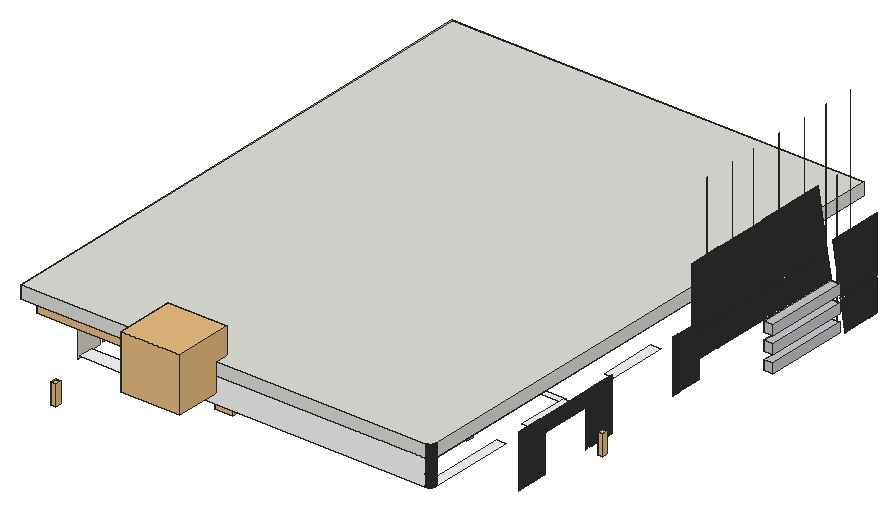
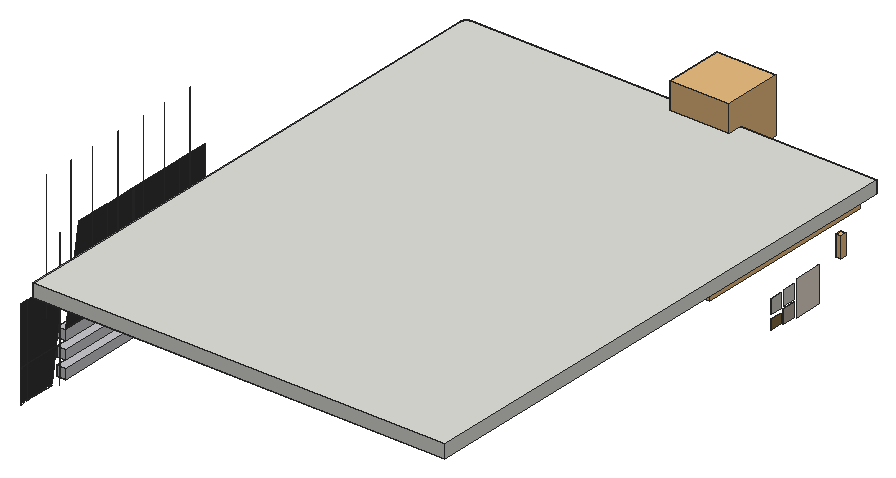
# SketchUp Ruby script. Lengths in inches.
U = 1.inch
M = Sketchup.active_model
def pt(a) = Geom::Point3d.new(a.map { |v| v * U })
def face(e, loops, mat)
  f = e.add_face(loops[0].map { |a| pt(a) })
  loops[1..].each { |l| e.add_face(l.map { |a| pt(a) }).erase! }
  f.material = f.back_material = mat if mat
  f
end
# faces: each face lists its corners as indices into pts; further lists are holes
def faces(e, pts, list, mat = nil) = list.each { |f| face(e, (f[0].is_a?(Array) ? f : [f]).map { |l| l.map { |i| pts[i] } }, mat) }
# xy, xz, yz: faces in a plane at the given z, y or x. An outline is a flat list of corners, or four numbers for a rectangle; further outlines are holes
def ring(l) = l.size == 4 ? [[l[0], l[1]], [l[2], l[1]], [l[2], l[3]], [l[0], l[3]]] : l.each_slice(2).to_a
def flat(e, list, mat, &to3) = list.each { |f| face(e, (f[0].is_a?(Array) ? f : [f]).map { |l| ring(l).map { |u, v| to3.(u, v) } }, mat) }
def xy(e, z, list, mat = nil) = flat(e, list, mat) { |x, y| [x, y, z] }
def xz(e, y, list, mat = nil) = flat(e, list, mat) { |x, z| [x, y, z] }
def yz(e, x, list, mat = nil) = flat(e, list, mat) { |y, z| [x, y, z] }
def lines(e, pts, list) = list.each { |a, b| e.add_line(pt(pts[a]), pt(pts[b])) }
# prism: a flat outline (further loops are holes) pulled along v
def prism(e, loops, v, mat = nil)
  f = face(e, loops, mat); d = Geom::Vector3d.new(v.map { |x| x * U })
  f.pushpull(f.normal.samedirection?(d) ? d.length : -d.length)
end
def box(e, o, s, mat = nil) = prism(e, [[o, [o[0] + s[0], o[1], o[2]], [o[0] + s[0], o[1] + s[1], o[2]], [o[0], o[1] + s[1], o[2]]]], [0, 0, s[2]], mat)
def at(x, y, z, deg = 0) = Geom::Transformation.translation(pt([x, y, z])) * Geom::Transformation.rotation(ORIGIN, Z_AXIS, deg.degrees)
def axes(o, x, y, z) = Geom::Transformation.new([*x, 0, *y, 0, *z, 0, *pt(o).to_a, 1])
def part(name) = M.definitions.add(name)
# library, detail: a bought-in or finely detailed component or shape, given as its bounding box
def library(name, o, s) = part(name).tap { |d| box(d.entities, o, s) }
def detail(e, o, s) = box(e.add_group.entities, o, s)
def put(e, d, t, mat = nil) = e.add_instance(d, t).tap { |i| i.material = mat if mat }
def group(e, t, mat = nil) = e.add_group.tap { |g| g.transformation = t; g.material = mat if mat }.entities
root = M.entities
M.materials.add("1513 AP K108 Rose Silver-N").color = [202, 201, 205]
M.materials.add("Laura_Hair").color = [160, 135, 94]
M.materials.add("Screenshot 2024-11-21 122829").color = [225, 216, 203]
M.materials.add("Screenshot 2024-11-21 123111").color = [210, 207, 202]
M.materials.add("Screenshot 2024-11-21 123347").color = [204, 201, 193]
M.materials.add("Screenshot 2024-11-21 123542").color = [178, 168, 157]
M.materials.add("Screenshot 2024-11-21 123654").color = [134, 109, 66]
M.materials.add("[0043_SaddleBrown]1").color = [139, 97, 33]
M.materials.add("[0047_Khaki]").color = [240, 230, 140]
M.materials.add("[0135_DarkGray]1").color = [81, 81, 81]
M.materials.add("[0136_Charcoal]").color = [35, 35, 35]
M.materials.add("[0137_Black]").color = [0, 0, 0]
M.materials.add("[Color D01]").color = [255, 242, 204]
M.materials.add("[Granite Dark Gray]").color = [51, 50, 50]
M.materials.add("[Quartz Light Grey]").color = [251, 251, 252]
c1 = library("UPLOAD",[122.71,32.39,0],[21.72,7.04,54.93])
c2 = part("4")
box(c2.entities,[0,-36,0],[9,78.24,9])
c3 = library("alu art",[7.69,0,0],[1.58,66.37,36.6])
c4 = part("Component\#78")
xy(c4.entities,0,[[0,0,6,9]],"Screenshot 2024-11-21 123347")
xy(c4.entities,1.5,[[0,0,6,9]],"Screenshot 2024-11-21 123347")
xz(c4.entities,0,[[0,0,6,1.5]],"[0047_Khaki]")
xz(c4.entities,9,[[0,0,6,1.5]],"[0047_Khaki]")
yz(c4.entities,0,[[0,0,9,1.5]],"[0047_Khaki]")
yz(c4.entities,6,[[0,0,9,1.5]],"[0047_Khaki]")
c5 = part("Component\#77")
xy(c5.entities,0,[[0,0,6,8]],"Screenshot 2024-11-21 123111")
xy(c5.entities,0.375,[[0,0,6,8]],"Screenshot 2024-11-21 123111")
xz(c5.entities,0,[[0,0,6,0.375]],"[0136_Charcoal]")
xz(c5.entities,8,[[0,0,6,0.375]],"[0136_Charcoal]")
yz(c5.entities,0,[[0,0,8,0.375]],"[0136_Charcoal]")
yz(c5.entities,6,[[0,0,8,0.375]],"[0136_Charcoal]")
c6 = part("Component\#76")
xy(c6.entities,0,[[0,0,24,36]],"Screenshot 2024-11-21 122829")
xy(c6.entities,0.7,[[0,0,24,36]],"Screenshot 2024-11-21 122829")
xz(c6.entities,0,[[0,0,24,0.7]],"[0135_DarkGray]1")
xz(c6.entities,36,[[0,0,24,0.7]],"[0135_DarkGray]1")
yz(c6.entities,0,[[0,0,36,0.7]],"[0135_DarkGray]1")
yz(c6.entities,24,[[0,0,36,0.7]],"[0135_DarkGray]1")
c7 = part("Component\#80")
xy(c7.entities,0,[[0,0,10,8]],"Screenshot 2024-11-21 123654")
xy(c7.entities,1.5,[[0,0,10,8]],"Screenshot 2024-11-21 123654")
xz(c7.entities,0,[[0,0,10,1.5]],"[0043_SaddleBrown]1")
xz(c7.entities,8,[[0,0,10,1.5]],"[0043_SaddleBrown]1")
yz(c7.entities,0,[[0,0,8,1.5]],"[0043_SaddleBrown]1")
yz(c7.entities,10,[[0,0,8,1.5]],"[0043_SaddleBrown]1")
c8 = part("Component\#79")
xy(c8.entities,0,[[0,0,6,6]],"Screenshot 2024-11-21 123542")
xy(c8.entities,1.5,[[0,0,6,6]],"Screenshot 2024-11-21 123542")
xz(c8.entities,0,[[0,0,6,1.5]],"[0137_Black]")
xz(c8.entities,6,[[0,0,6,1.5]],"[0137_Black]")
yz(c8.entities,0,[[0,0,6,1.5]],"[0137_Black]")
yz(c8.entities,6,[[0,0,6,1.5]],"[0137_Black]")
c9 = part("wallart")
g1 = group(c9.entities,at(0,0,0))
put(g1,c4,axes([44.59,0,15.65],[1.7388,0,0],[0,0,1.4322],[0,-0.42,0]))
put(g1,c5,axes([29.35,0,16.47],[1.9152,0,0],[0,0,1.68],[0,-1.68,0]))
put(g1,c6,axes([0,0,0],[1.06957,0,0],[0,0,0.8988],[0,-0.8988,0]),"[0136_Charcoal]")
put(g1,c7,axes([45.17,0,2.94],[1.05,0,0],[0,0,1.1046],[0,-0.42,0]))
put(g1,c8,axes([28.96,0,1.29],[2.0328,0,0],[0,0,2.1],[0,-0.42,0]))
c10 = library("WALL LIGHT 69",[4.19,4.05,-9.63],[4.61,5.7,18.83])
c11 = library("Group\#103",[0,0,0],[31.5,31.5,74.4])
c12 = library("Group\#95",[0,0,0],[31.5,31.5,74.4])
c13 = library("Group\#83",[0,0,0],[31.5,31.5,74.4])
c14 = library("Group\#86",[0,0,0],[31.5,31.5,74.4])
c15 = library("Group\#85",[0,0,0],[31.5,31.5,74.4])
c16 = library("Group\#118",[0,0,0],[31.5,31.5,74.4])
c17 = part("Plant Wall Art")
g2 = group(c17.entities,at(1.72,0.59,0))
xy(g2,0,[[0,-0.59,13.78,0]],"Laura_Hair")
xy(g2,0.39,[[0.39,-0.59,13.39,-0.39]],"Laura_Hair")
xy(g2,19.29,[[0.39,-0.59,13.39,-0.39]],"Laura_Hair")
xy(g2,19.69,[[0,-0.59,13.78,0]],"Laura_Hair")
xz(g2,-0.59,[[[0,0,13.78,19.69],[0.39,0.39,13.39,19.29]]],"Laura_Hair")
xz(g2,0,[[0,0,13.78,19.69]],"Laura_Hair")
yz(g2,0,[[-0.59,0,0,19.69]],"Laura_Hair")
yz(g2,0.39,[[-0.59,0.39,-0.39,19.29]],"Laura_Hair")
yz(g2,13.39,[[-0.59,0.39,-0.39,19.29]],"Laura_Hair")
yz(g2,13.78,[[-0.59,0,0,19.69]],"Laura_Hair")
p = [[13.39,0,0.39],[13.39,-0.39,0.39],[13.39,0,19.29],[13.39,-0.39,19.29],[0.39,0,0.39],[0.39,-0.39,0.39],
  [0.39,0,19.29],[0.39,-0.39,19.29]]
lines(g2,p,[[0,1],[2,3],[4,5],[6,7]])
g3 = group(c17.entities,at(19.43,0.59,0))
xy(g3,0,[[0,-0.59,13.78,0]],"Laura_Hair")
xy(g3,0.39,[[0.39,-0.59,13.39,-0.39]],"Laura_Hair")
xy(g3,19.29,[[0.39,-0.59,13.39,-0.39]],"Laura_Hair")
xy(g3,19.69,[[0,-0.59,13.78,0]],"Laura_Hair")
xz(g3,-0.59,[[[0,0,13.78,19.69],[0.39,0.39,13.39,19.29]]],"Laura_Hair")
xz(g3,0,[[0,0,13.78,19.69]],"Laura_Hair")
yz(g3,0,[[-0.59,0,0,19.69]],"Laura_Hair")
yz(g3,0.39,[[-0.59,0.39,-0.39,19.29]],"Laura_Hair")
yz(g3,13.39,[[-0.59,0.39,-0.39,19.29]],"Laura_Hair")
yz(g3,13.78,[[-0.59,0,0,19.69]],"Laura_Hair")
p = [[13.39,0,0.39],[13.39,-0.39,0.39],[13.39,0,19.29],[13.39,-0.39,19.29],[0.39,0,0.39],[0.39,-0.39,0.39],
  [0.39,0,19.29],[0.39,-0.39,19.29]]
lines(g3,p,[[0,1],[2,3],[4,5],[6,7]])
g4 = group(c17.entities,at(37.15,0.59,0))
xy(g4,0,[[0,-0.59,13.78,0]],"Laura_Hair")
xy(g4,0.39,[[0.39,-0.59,13.39,-0.39]],"Laura_Hair")
xy(g4,19.29,[[0.39,-0.59,13.39,-0.39]],"Laura_Hair")
xy(g4,19.69,[[0,-0.59,13.78,0]],"Laura_Hair")
xz(g4,-0.59,[[[0,0,13.78,19.69],[0.39,0.39,13.39,19.29]]],"Laura_Hair")
xz(g4,0,[[0,0,13.78,19.69]],"Laura_Hair")
yz(g4,0,[[-0.59,0,0,19.69]],"Laura_Hair")
yz(g4,0.39,[[-0.59,0.39,-0.39,19.29]],"Laura_Hair")
yz(g4,13.39,[[-0.59,0.39,-0.39,19.29]],"Laura_Hair")
yz(g4,13.78,[[-0.59,0,0,19.69]],"Laura_Hair")
p = [[13.39,0,0.39],[13.39,-0.39,0.39],[13.39,0,19.29],[13.39,-0.39,19.29],[0.39,0,0.39],[0.39,-0.39,0.39],
  [0.39,0,19.29],[0.39,-0.39,19.29]]
lines(g4,p,[[0,1],[2,3],[4,5],[6,7]])
c18 = library("Potted trailing plant",[-13.52,-13.75,-7.41],[40.56,40.5625,37.31])
c19 = library("Group\#499",[0,24,0],[134.36,119.61,16.18])
xy(root,164,[[443.875,563.39,444,591],[443.875,592,444,600]],"[Granite Dark Gray]")
xy(root,165,[[443.875,563.22,444,591],[443.875,592,444,600]],"[Granite Dark Gray]")
xy(root,194,[[443.875,558.17,444,591],[443.875,592,444,600]],"[Granite Dark Gray]")
xy(root,195,[[443.875,558,444,591],[443.875,592,444,600]],"[Granite Dark Gray]")
xy(root,199,[[443.875,183,444,207],[443.875,208,444,213],[443.875,261,444,267],[443.875,268,444,291],[443.875,363,444,369],
  [443.875,370,444,393]],"[Granite Dark Gray]")
xy(root,200,[[443.875,183,444,207],[443.875,208,444,213],[443.875,261,444,267],[443.875,268,444,291],[443.875,363,444,369],
  [443.875,370,444,393]],"[Granite Dark Gray]")
xy(root,210,[[436.875,393,437,423],[436.875,424,437,477],[436.875,478,437,507],[436.875,508,437,555.39]],"[Granite Dark Gray]")
xy(root,211,[[436.875,393,437,423],[436.875,424,437,477],[436.875,478,437,507],[436.875,508,437,555.22]],"[Granite Dark Gray]")
xy(root,222,[[351,273,411,279]],"[Quartz Light Grey]")
xy(root,234,[[432,213,444,261],[436.875,393,437,423],[436.875,424,437,477],[436.875,478,437,507],[436.875,508,437,551.22]],"[Granite Dark Gray]")
xy(root,234,[[108,90,156,105],[180,96,180,105,423,105,423,183,432,183,432,101.78,431.95,101.23,431.93,101.12,431.92,101.01,431.9,100.9,431.85,100.68,431.83,100.57,431.8,100.46,431.77,100.36,431.74,100.25,431.71,100.15,431.67,100.04,431.63,99.9375,431.59,99.83,431.47,99.53,431.27,99.13,431.21,99.03,431.16,98.9375,431.1,98.84,430.98,98.66,430.92,98.5625,430.85,98.47,430.79,98.38,430.72,98.3,430.65,98.21,430.51,98.04,430.43,97.96,430.36,97.875,430.28,97.8,430.2,97.72,430.125,97.64,430.04,97.57,429.96,97.49,429.79,97.35,429.7,97.28,429.62,97.21,429.53,97.15,429.4375,97.08,429.34,97.02,429.16,96.9,429.0625,96.84,428.97,96.79,428.87,96.73,428.47,96.53,428.17,96.41,428.0625,96.37,427.96,96.33,427.85,96.29,427.75,96.26,427.64,96.23,427.54,96.2,427.43,96.17,427.32,96.15,427.1,96.1,426.99,96.08,426.88,96.07,426.77,96.05,426.22,96],[423,213,432,261],[423,309,432,363]],"[Quartz Light Grey]")
xy(root,235,[[436.875,393,437,423],[436.875,424,437,477],[436.875,478,437,507],[436.875,508,437,551.04]],"[Granite Dark Gray]")
xz(root,96,[[180,234,426,258],[426,234,426.11,258],[426.11,234,426.22,258]],"[Quartz Light Grey]")
xz(root,207,[[443.875,200,444,248]],"[Granite Dark Gray]")
xz(root,208,[[443.875,200,444,248]],"[Granite Dark Gray]")
xz(root,267,[[443.875,200,444,248]],"[Granite Dark Gray]")
xz(root,268,[[443.875,200,444,248]],"[Granite Dark Gray]")
xz(root,369,[[443.875,200,444,248]],"[Granite Dark Gray]")
xz(root,370,[[443.875,200,444,248]],"[Granite Dark Gray]")
xz(root,423,[[436.875,211,437,234],[436.875,235,437,294]],"[Granite Dark Gray]")
xz(root,424,[[436.875,211,437,234],[436.875,235,437,294]],"[Granite Dark Gray]")
xz(root,477,[[436.875,211,437,234],[436.875,235,437,294]],"[Granite Dark Gray]")
xz(root,478,[[436.875,211,437,234],[436.875,235,437,294]],"[Granite Dark Gray]")
xz(root,507,[[436.875,211,437,234],[436.875,235,437,294]],"[Granite Dark Gray]")
xz(root,508,[[436.875,211,437,234],[436.875,235,437,294]],"[Granite Dark Gray]")
xz(root,591,[[443.875,165,444,194],[443.875,195,444,199],[443.875,199,444,200],[443.875,200,444,248]],"[Granite Dark Gray]")
xz(root,592,[[443.875,165,444,194],[443.875,195,444,199],[443.875,199,444,200],[443.875,200,444,248]],"[Granite Dark Gray]")
yz(root,432,[[101.78,234,101.89,258],[101.89,234,102,258]],"[Quartz Light Grey]")
yz(root,437,[[393,211,423,234],[424,211,477,234],[478,211,507,234],[508,211,555.22,211,551.22,234,508,234],[393,235,423,294],
  [424,235,477,294],[478,235,507,294],[508,235,551.04,235,540.78,294,508,294]],"[Granite Dark Gray]")
yz(root,444,[[563.22,165,591,165,591,194,558.17,194],[592,165,600,194],[558,195,591,195,591,248,548.78,248],[592,195,600,248],[183,200,207,248],
  [208,200,213,200,213,234,261,234,261,200,267,200,267,248,208,248],[268,200,291,248],[363,200,369,248],[370,200,393,248]],"[Granite Dark Gray]")
p = [[426.33,96.01,258],[426.22,96,258],[426.22,96,234],[426.33,96.01,234],[426.44,96.02,258],[426.44,96.02,234],
  [426.55,96.03,258],[426.55,96.03,234],[426.66,96.04,258],[426.66,96.04,234],[426.77,96.05,258],[426.77,96.05,234],
  [426.88,96.07,258],[426.88,96.07,234],[426.99,96.08,258],[426.99,96.08,234],[427.1,96.1,258],[427.1,96.1,234],
  [427.21,96.125,258],[427.21,96.125,234],[427.32,96.15,258],[427.32,96.15,234],[427.43,96.17,258],[427.43,96.17,234],
  [427.54,96.2,258],[427.54,96.2,234],[427.64,96.23,258],[427.64,96.23,234],[427.75,96.26,258],[427.75,96.26,234],
  [427.85,96.29,258],[427.85,96.29,234],[427.96,96.33,258],[427.96,96.33,234],[428.0625,96.37,258],[428.0625,96.37,234],
  [428.17,96.41,258],[428.17,96.41,234],[428.27,96.45,258],[428.27,96.45,234],[428.37,96.49,258],[428.37,96.49,234],
  [428.47,96.53,258],[428.47,96.53,234],[428.57,96.58,258],[428.57,96.58,234],[428.67,96.63,258],[428.67,96.63,234],
  [428.77,96.68,258],[428.77,96.68,234],[428.87,96.73,258],[428.87,96.73,234],[428.97,96.79,258],[428.97,96.79,234],
  [429.0625,96.84,258],[429.0625,96.84,234],[429.16,96.9,258],[429.16,96.9,234],[429.25,96.96,258],[429.25,96.96,234],
  [429.4375,97.08,258],[429.34,97.02,258],[429.34,97.02,234],[429.4375,97.08,234],[429.53,97.15,258],[429.53,97.15,234],
  [429.62,97.21,258],[429.62,97.21,234],[429.7,97.28,258],[429.7,97.28,234],[429.79,97.35,258],[429.79,97.35,234],
  [429.875,97.42,258],[429.875,97.42,234],[429.96,97.49,258],[429.96,97.49,234],[430.04,97.57,258],[430.04,97.57,234],
  [430.125,97.64,258],[430.125,97.64,234],[430.2,97.72,258],[430.2,97.72,234],[430.28,97.8,258],[430.28,97.8,234],
  [430.36,97.875,258],[430.36,97.875,234],[430.43,97.96,258],[430.43,97.96,234],[430.51,98.04,258],[430.51,98.04,234],
  [430.58,98.125,258],[430.58,98.125,234],[430.65,98.21,258],[430.65,98.21,234],[430.72,98.3,258],[430.72,98.3,234],
  [430.79,98.38,258],[430.79,98.38,234],[430.85,98.47,258],[430.85,98.47,234],[430.92,98.5625,258],[430.92,98.5625,234],
  [430.98,98.66,258],[430.98,98.66,234],[431.04,98.75,258],[431.04,98.75,234],[431.1,98.84,258],[431.1,98.84,234],
  [431.16,98.9375,258],[431.16,98.9375,234],[431.21,99.03,258],[431.21,99.03,234],[431.27,99.13,258],[431.27,99.13,234],
  [431.32,99.23,258],[431.32,99.23,234],[431.37,99.33,258],[431.37,99.33,234],[431.42,99.43,258],[431.42,99.43,234],
  [431.47,99.53,258],[431.47,99.53,234],[431.51,99.63,258],[431.51,99.63,234],[431.55,99.73,258],[431.55,99.73,234],
  [431.59,99.83,258],[431.59,99.83,234],[431.63,99.9375,258],[431.63,99.9375,234],[431.67,100.04,258],[431.67,100.04,234],
  [431.71,100.15,258],[431.71,100.15,234],[431.74,100.25,258],[431.74,100.25,234],[431.77,100.36,258],[431.77,100.36,234],
  [431.8,100.46,258],[431.8,100.46,234],[431.83,100.57,258],[431.83,100.57,234],[431.85,100.68,258],[431.85,100.68,234],
  [431.875,100.79,258],[431.875,100.79,234],[431.9,100.9,258],[431.9,100.9,234],[431.92,101.01,258],[431.92,101.01,234],
  [431.93,101.12,258],[431.93,101.12,234],[431.95,101.23,258],[431.95,101.23,234],[431.96,101.34,258],[431.96,101.34,234],
  [431.97,101.45,258],[431.97,101.45,234],[431.98,101.56,258],[431.98,101.56,234],[431.99,101.67,258],[431.99,101.67,234],
  [432,101.78,258],[432,101.78,234],[432,417,234],[432,417,354],[432,447,234],[432,447,235],
  [432,531,234],[432,531,354],[432,585,234],[432,585,354],[437,555.39,211],[437,555.22,211],
  [432,447,354],[437,551.04,235],[437,551.22,235],[432,418,234],[432,418,354],[432,471,234],
  [432,471,354],[432,472,234],[432,472,354],[432,501,234],[432,501,354],[432,502,234],
  [432,502,354],[432,556,234],[432,556,354],[437,562,294],[437,562,235],[437,562,234],
  [437,562,211],[437,562,210],[437,562,172],[437,563,172],[437,563,166.25],[437,563,234],
  [437,563,211],[437,563,210],[437,563,294],[437,563,235],[432,557,234],[432,557,354]]
faces(root,p,[[0,1,2,3],[4,0,3,5],[6,4,5,7],[8,6,7,9],[10,8,9,11],[12,10,11,13],[14,12,13,15],[16,14,15,17],
  [18,16,17,19],[20,18,19,21],[22,20,21,23],[24,22,23,25],[26,24,25,27],[28,26,27,29],[30,28,29,31],[32,30,31,33],
  [34,32,33,35],[36,34,35,37],[38,36,37,39],[40,38,39,41],[42,40,41,43],[44,42,43,45],[46,44,45,47],[48,46,47,49],
  [50,48,49,51],[52,50,51,53],[54,52,53,55],[56,54,55,57],[58,56,57,59],[60,61,62,63],[61,58,59,62],[64,60,63,65],
  [66,64,65,67],[68,66,67,69],[70,68,69,71],[72,70,71,73],[74,72,73,75],[76,74,75,77],[78,76,77,79],[80,78,79,81],
  [82,80,81,83],[84,82,83,85],[86,84,85,87],[88,86,87,89],[90,88,89,91],[92,90,91,93],[94,92,93,95],[96,94,95,97],
  [98,96,97,99],[100,98,99,101],[102,100,101,103],[104,102,103,105],[106,104,105,107],[108,106,107,109],[110,108,109,111],[112,110,111,113],
  [114,112,113,115],[116,114,115,117],[118,116,117,119],[120,118,119,121],[122,120,121,123],[124,122,123,125],[126,124,125,127],[128,126,127,129],
  [130,128,129,131],[132,130,131,133],[134,132,133,135],[136,134,135,137],[138,136,137,139],[140,138,139,141],[142,140,141,143],[144,142,143,145],
  [146,144,145,147],[148,146,147,149],[150,148,149,151],[152,150,151,153],[154,152,153,155],[156,154,155,157],[158,156,157,159],[160,158,159,161],
  [162,160,161,163]],"[Quartz Light Grey]")
lines(root,p,[[164,165],[166,167],[168,169],[170,171],[172,173],[167,174],[175,176],[177,178],[179,180],[181,182],[183,184],[185,186],
  [187,188],[189,190],[191,192],[193,194],[195,196],[197,198],[199,195],[200,201],[202,203]])
put(root,c1,at(72.42,233.57,163.4),"[Quartz Light Grey]")
put(root,c1,axes([451.66,233.57,163.4],[-1,0,0],[0,1,0],[0,0,1]),"[Quartz Light Grey]")
put(root,c2,at(437,513,168),"1513 AP K108 Rose Silver-N")
put(root,c3,axes([222.73,281.39,168],[0,-1.188,0],[1.188,0,0],[0,0,1.188]),"[Quartz Light Grey]")
put(root,c2,at(437,513,184),"1513 AP K108 Rose Silver-N")
put(root,c9,at(57,151.57,187.28,90),"[Quartz Light Grey]")
put(root,c10,at(81.74,80.25,197.85))
put(root,c10,at(439.81,270.49,198.43))
put(root,c2,at(437,513,200),"1513 AP K108 Rose Silver-N")
put(root,c11,axes([257.73,193.36,209.25],[0.53882,0,0],[0,0.41681,0],[0,0,0.588]),"[Color D01]")
put(root,c12,axes([257.73,147.71,209.25],[0.53882,0,0],[0,0.41681,0],[0,0,0.588]),"[Color D01]")
put(root,c13,axes([348.77,228.92,209.25],[0.53882,0,0],[0,0.41681,0],[0,0,0.588]),"[Color D01]")
put(root,c14,axes([348.77,183.28,209.25],[0.53882,0,0],[0,0.41681,0],[0,0,0.588]),"[Color D01]")
put(root,c15,axes([206.63,124.89,209.25],[0.53882,0,0],[0,0.41681,0],[0,0,0.588]),"[Color D01]")
put(root,c16,axes([223.66,239,209.25],[0.53882,0,0],[0,0.41681,0],[0,0,0.588]),"[Color D01]")
put(root,c17,at(172.72,162.07,223.73,90),"[Quartz Light Grey]")
put(root,c18,axes([193.82,72.43,253.67],[1.36,0,0],[0,1.36,0],[0,0,1.36]))
g5 = group(root,at(57,105,270))
xy(g5,-12,[[[-9,-9,-9,495,375,495,375,-3.22,374.95,-3.77,374.93,-3.88,374.92,-3.99,374.9,-4.1,374.85,-4.32,374.83,-4.43,374.8,-4.54,374.77,-4.64,374.74,-4.75,374.71,-4.85,374.67,-4.96,374.63,-5.0625,374.59,-5.17,374.47,-5.47,374.27,-5.87,374.21,-5.97,374.16,-6.0625,374.1,-6.16,373.98,-6.34,373.92,-6.4375,373.85,-6.53,373.79,-6.62,373.72,-6.7,373.65,-6.79,373.51,-6.96,373.43,-7.04,373.36,-7.125,373.28,-7.2,373.2,-7.28,373.125,-7.36,373.04,-7.43,372.96,-7.51,372.79,-7.65,372.7,-7.72,372.62,-7.79,372.53,-7.85,372.4375,-7.92,372.34,-7.98,372.16,-8.1,372.0625,-8.16,371.97,-8.21,371.87,-8.27,371.47,-8.47,371.17,-8.59,371.0625,-8.63,370.96,-8.67,370.85,-8.71,370.75,-8.74,370.64,-8.77,370.54,-8.8,370.43,-8.83,370.32,-8.85,370.1,-8.9,369.99,-8.92,369.88,-8.93,369.77,-8.95,369.22,-9],[114,0,366,168],[0,0,108,174]]])
xy(g5,-6,[[0,0,108,174],[114,0,366,168]])
xy(g5,0,[[-9,-9,369.22,-9,369.77,-8.95,369.88,-8.93,369.99,-8.92,370.1,-8.9,370.32,-8.85,370.43,-8.83,370.54,-8.8,370.64,-8.77,370.75,-8.74,370.85,-8.71,370.96,-8.67,371.0625,-8.63,371.17,-8.59,371.47,-8.47,371.87,-8.27,371.97,-8.21,372.0625,-8.16,372.16,-8.1,372.34,-7.98,372.4375,-7.92,372.53,-7.85,372.62,-7.79,372.7,-7.72,372.79,-7.65,372.96,-7.51,373.04,-7.43,373.125,-7.36,373.2,-7.28,373.28,-7.2,373.36,-7.125,373.43,-7.04,373.51,-6.96,373.65,-6.79,373.72,-6.7,373.79,-6.62,373.85,-6.53,373.92,-6.4375,373.98,-6.34,374.1,-6.16,374.16,-6.0625,374.21,-5.97,374.27,-5.87,374.47,-5.47,374.59,-5.17,374.63,-5.0625,374.67,-4.96,374.71,-4.85,374.74,-4.75,374.77,-4.64,374.8,-4.54,374.83,-4.43,374.85,-4.32,374.9,-4.1,374.92,-3.99,374.93,-3.88,374.95,-3.77,375,-3.22,375,495,-9,495]])
xz(g5,-9,[[-9,-12,369,0],[369,-12,369.11,0],[369.11,-12,369.22,0]])
xz(g5,0,[[0,-12,108,-6],[114,-12,366,-6]])
xz(g5,168,[[114,-12,366,-6]])
xz(g5,174,[[0,-12,108,-6]])
xz(g5,495,[[-9,-12,375,0]])
yz(g5,-9,[[-9,-12,495,0]])
yz(g5,0,[[0,-12,174,-6]])
yz(g5,108,[[0,-12,168,-6],[168,-12,174,-6]])
yz(g5,114,[[0,-12,168,-6]])
yz(g5,366,[[0,-12,168,-6]])
yz(g5,375,[[-3.22,-12,-3.11,0],[-3.11,-12,-3,0],[-3,-12,495,0]])
p = [[369.33,-8.99,0],[369.22,-9,0],[369.22,-9,-12],[369.33,-8.99,-12],[369.44,-8.98,0],[369.44,-8.98,-12],
  [369.55,-8.97,0],[369.55,-8.97,-12],[369.66,-8.96,0],[369.66,-8.96,-12],[369.77,-8.95,0],[369.77,-8.95,-12],
  [369.88,-8.93,0],[369.88,-8.93,-12],[369.99,-8.92,0],[369.99,-8.92,-12],[370.1,-8.9,0],[370.1,-8.9,-12],
  [370.21,-8.875,0],[370.21,-8.875,-12],[370.32,-8.85,0],[370.32,-8.85,-12],[370.43,-8.83,0],[370.43,-8.83,-12],
  [370.54,-8.8,0],[370.54,-8.8,-12],[370.64,-8.77,0],[370.64,-8.77,-12],[370.75,-8.74,0],[370.75,-8.74,-12],
  [370.85,-8.71,0],[370.85,-8.71,-12],[370.96,-8.67,0],[370.96,-8.67,-12],[371.0625,-8.63,0],[371.0625,-8.63,-12],
  [371.17,-8.59,0],[371.17,-8.59,-12],[371.27,-8.55,0],[371.27,-8.55,-12],[371.37,-8.51,0],[371.37,-8.51,-12],
  [371.47,-8.47,0],[371.47,-8.47,-12],[371.57,-8.42,0],[371.57,-8.42,-12],[371.67,-8.37,0],[371.67,-8.37,-12],
  [371.77,-8.32,0],[371.77,-8.32,-12],[371.87,-8.27,0],[371.87,-8.27,-12],[371.97,-8.21,0],[371.97,-8.21,-12],
  [372.0625,-8.16,0],[372.0625,-8.16,-12],[372.16,-8.1,0],[372.16,-8.1,-12],[372.25,-8.04,0],[372.25,-8.04,-12],
  [372.4375,-7.92,0],[372.34,-7.98,0],[372.34,-7.98,-12],[372.4375,-7.92,-12],[372.53,-7.85,0],[372.53,-7.85,-12],
  [372.62,-7.79,0],[372.62,-7.79,-12],[372.7,-7.72,0],[372.7,-7.72,-12],[372.79,-7.65,0],[372.79,-7.65,-12],
  [372.875,-7.58,0],[372.875,-7.58,-12],[372.96,-7.51,0],[372.96,-7.51,-12],[373.04,-7.43,0],[373.04,-7.43,-12],
  [373.125,-7.36,0],[373.125,-7.36,-12],[373.2,-7.28,0],[373.2,-7.28,-12],[373.28,-7.2,0],[373.28,-7.2,-12],
  [373.36,-7.125,0],[373.36,-7.125,-12],[373.43,-7.04,0],[373.43,-7.04,-12],[373.51,-6.96,0],[373.51,-6.96,-12],
  [373.58,-6.875,0],[373.58,-6.875,-12],[373.65,-6.79,0],[373.65,-6.79,-12],[373.72,-6.7,0],[373.72,-6.7,-12],
  [373.79,-6.62,0],[373.79,-6.62,-12],[373.85,-6.53,0],[373.85,-6.53,-12],[373.92,-6.4375,0],[373.92,-6.4375,-12],
  [373.98,-6.34,0],[373.98,-6.34,-12],[374.1,-6.16,0],[374.04,-6.25,0],[374.04,-6.25,-12],[374.1,-6.16,-12],
  [374.16,-6.0625,0],[374.16,-6.0625,-12],[374.21,-5.97,0],[374.21,-5.97,-12],[374.27,-5.87,0],[374.27,-5.87,-12],
  [374.32,-5.77,0],[374.32,-5.77,-12],[374.37,-5.67,0],[374.37,-5.67,-12],[374.42,-5.57,0],[374.42,-5.57,-12],
  [374.47,-5.47,0],[374.47,-5.47,-12],[374.51,-5.37,0],[374.51,-5.37,-12],[374.55,-5.27,0],[374.55,-5.27,-12],
  [374.59,-5.17,0],[374.59,-5.17,-12],[374.63,-5.0625,0],[374.63,-5.0625,-12],[374.67,-4.96,0],[374.67,-4.96,-12],
  [374.71,-4.85,0],[374.71,-4.85,-12],[374.74,-4.75,0],[374.74,-4.75,-12],[374.77,-4.64,0],[374.77,-4.64,-12],
  [374.8,-4.54,0],[374.8,-4.54,-12],[374.83,-4.43,0],[374.83,-4.43,-12],[374.85,-4.32,0],[374.85,-4.32,-12],
  [374.875,-4.21,0],[374.875,-4.21,-12],[374.9,-4.1,0],[374.9,-4.1,-12],[374.92,-3.99,0],[374.92,-3.99,-12],
  [374.93,-3.88,0],[374.93,-3.88,-12],[374.95,-3.77,0],[374.95,-3.77,-12],[374.96,-3.66,0],[374.96,-3.66,-12],
  [374.97,-3.55,0],[374.97,-3.55,-12],[374.98,-3.44,0],[374.98,-3.44,-12],[374.99,-3.33,0],[374.99,-3.33,-12],
  [375,-3.22,0],[375,-3.22,-12],[114,168,-12],[114,174,-12]]
faces(g5,p,[[0,1,2,3],[4,0,3,5],[6,4,5,7],[8,6,7,9],[10,8,9,11],[12,10,11,13],[14,12,13,15],[16,14,15,17],
  [18,16,17,19],[20,18,19,21],[22,20,21,23],[24,22,23,25],[26,24,25,27],[28,26,27,29],[30,28,29,31],[32,30,31,33],
  [34,32,33,35],[36,34,35,37],[38,36,37,39],[40,38,39,41],[42,40,41,43],[44,42,43,45],[46,44,45,47],[48,46,47,49],
  [50,48,49,51],[52,50,51,53],[54,52,53,55],[56,54,55,57],[58,56,57,59],[60,61,62,63],[61,58,59,62],[64,60,63,65],
  [66,64,65,67],[68,66,67,69],[70,68,69,71],[72,70,71,73],[74,72,73,75],[76,74,75,77],[78,76,77,79],[80,78,79,81],
  [82,80,81,83],[84,82,83,85],[86,84,85,87],[88,86,87,89],[90,88,89,91],[92,90,91,93],[94,92,93,95],[96,94,95,97],
  [98,96,97,99],[100,98,99,101],[102,100,101,103],[104,105,106,107],[105,102,103,106],[108,104,107,109],[110,108,109,111],[112,110,111,113],
  [114,112,113,115],[116,114,115,117],[118,116,117,119],[120,118,119,121],[122,120,121,123],[124,122,123,125],[126,124,125,127],[128,126,127,129],
  [130,128,129,131],[132,130,131,133],[134,132,133,135],[136,134,135,137],[138,136,137,139],[140,138,139,141],[142,140,141,143],[144,142,143,145],
  [146,144,145,147],[148,146,147,149],[150,148,149,151],[152,150,151,153],[154,152,153,155],[156,154,155,157],[158,156,157,159],[160,158,159,161],
  [162,160,161,163]])
lines(g5,p,[[164,165]])
put(g5,c19,axes([-21.67,174,-24.24],[0,-1.29988,0],[0.90296,0,0],[0,0,1]))
